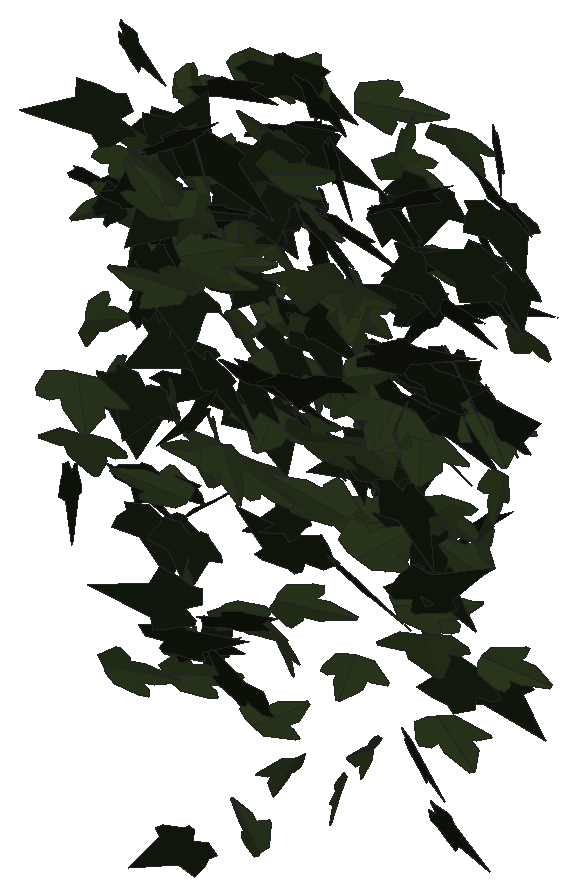
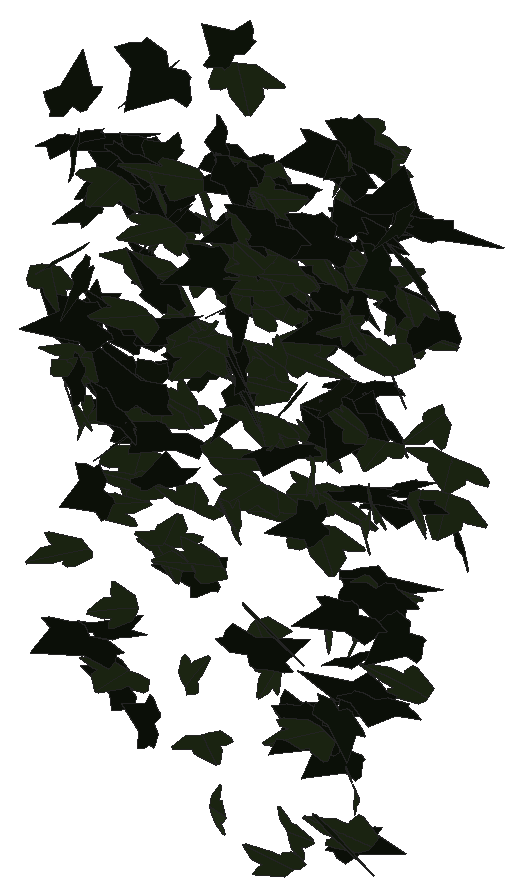
# SketchUp Ruby script. Lengths in millimetres.
U = 1.mm
M = Sketchup.active_model
def pt(a) = Geom::Point3d.new(a.map { |v| v * U })
def face(e, loops, mat)
  f = e.add_face(loops[0].map { |a| pt(a) })
  loops[1..].each { |l| e.add_face(l.map { |a| pt(a) }).erase! }
  f.material = f.back_material = mat if mat
  f
end
# faces: each face lists its corners as indices into pts; further lists are holes
def faces(e, pts, list, mat = nil) = list.each { |f| face(e, (f[0].is_a?(Array) ? f : [f]).map { |l| l.map { |i| pts[i] } }, mat) }
# xy, xz, yz: faces in a plane at the given z, y or x. An outline is a flat list of corners, or four numbers for a rectangle; further outlines are holes
def ring(l) = l.size == 4 ? [[l[0], l[1]], [l[2], l[1]], [l[2], l[3]], [l[0], l[3]]] : l.each_slice(2).to_a
def flat(e, list, mat, &to3) = list.each { |f| face(e, (f[0].is_a?(Array) ? f : [f]).map { |l| ring(l).map { |u, v| to3.(u, v) } }, mat) }
def xy(e, z, list, mat = nil) = flat(e, list, mat) { |x, y| [x, y, z] }
def xz(e, y, list, mat = nil) = flat(e, list, mat) { |x, z| [x, y, z] }
def yz(e, x, list, mat = nil) = flat(e, list, mat) { |y, z| [x, y, z] }
def lines(e, pts, list) = list.each { |a, b| e.add_line(pt(pts[a]), pt(pts[b])) }
# prism: a flat outline (further loops are holes) pulled along v
def prism(e, loops, v, mat = nil)
  f = face(e, loops, mat); d = Geom::Vector3d.new(v.map { |x| x * U })
  f.pushpull(f.normal.samedirection?(d) ? d.length : -d.length)
end
def box(e, o, s, mat = nil) = prism(e, [[o, [o[0] + s[0], o[1], o[2]], [o[0] + s[0], o[1] + s[1], o[2]], [o[0], o[1] + s[1], o[2]]]], [0, 0, s[2]], mat)
def at(x, y, z, deg = 0) = Geom::Transformation.translation(pt([x, y, z])) * Geom::Transformation.rotation(ORIGIN, Z_AXIS, deg.degrees)
def axes(o, x, y, z) = Geom::Transformation.new([*x, 0, *y, 0, *z, 0, *pt(o).to_a, 1])
def part(name) = M.definitions.add(name)
# library, detail: a bought-in or finely detailed component or shape, given as its bounding box
def library(name, o, s) = part(name).tap { |d| box(d.entities, o, s) }
def detail(e, o, s) = box(e.add_group.entities, o, s)
def put(e, d, t, mat = nil) = e.add_instance(d, t).tap { |i| i.material = mat if mat }
def group(e, t, mat = nil) = e.add_group.tap { |g| g.transformation = t; g.material = mat if mat }.entities
root = M.entities
M.materials.add("efeu1").color = [18, 25, 13]
M.materials.add("efeu2").color = [43, 57, 29]
c1 = part("ivyleaf_9")
p = [[39.1,54.8,31.7],[34.5,51.8,30.2],[-5.3,25.2,17.3],[-17.9,28.3,20.9],[-21.6,21.7,17],[-20.2,4.3,5.3],
  [-22.9,-0.3,2.5],[-17.1,-4,-0.6],[-2,-2.1,-1.2],[-0.7,-15.4,-10.1],[16.6,-22.3,-16.7],[21.1,-15.1,-12.5],
  [32.7,-10.7,-11],[46.1,-1.8,-6.6],[30.8,11.2,3.8]]
faces(c1.entities,p,[[0,1,2,3,4,5,6,7,8,9,10,11,12,13,14]],"efeu1")
c2 = part("ivyleaf_10")
p = [[0,12.8,-0.8],[-1.5,51.3,-10.9],[-4.9,51,-11.6],[-13.6,26.5,-7.3],[-13.2,15.9,-4.6],[-21.1,19.3,-7.2],
  [-29.5,16.3,-8.3],[-29.2,8.3,-6.2],[-19.7,-9.8,0.5],[-7.6,-13,4],[1,-12.2,5.8],[-0.4,51.1,-11.1],
  [-1.5,51.1,-10.9],[1,-12.4,5.9],[16.9,-12.4,3.5],[35.1,9.1,-5.1],[35,12.9,-6.1],[20.5,16.4,-4.9],
  [15.8,15,-3.8],[15.3,27.6,-7.1],[12.8,31.3,-7.8]]
faces(c2.entities,p,[[0,1,2,3,4,5,6,7,8,9,10],[11,12,0,13,14,15,16,17,18,19,20]],"efeu2")
put(root,c1,axes([4369.1,966.1,860.8],[0.08362,0.95421,0.22388],[0.01446,0.22376,-0.95522],[-1.86531,0.04451,0.00263]))
put(root,c1,axes([4349,904.5,861.4],[-1.16613,-0.65303,-0.50074],[0.6447,0.3688,-0.89547],[1.42733,-0.70011,-0.00464]))
put(root,c1,axes([4339.9,842.3,951.2],[1.8565,-0.13492,-0.2079],[-0.3923,0.02714,-0.98475],[0.26191,0.997,-0.00132]))
put(root,c2,axes([4325.6,979.6,1366.4],[0.13539,-0.04871,-0.98589],[1.45694,-0.62129,0.08593],[-1.18599,-0.76879,-0.00698]))
put(root,c1,axes([4331.7,974.3,1044],[-0.12536,-0.06032,-0.97559],[1.05105,0.80448,-0.08703],[1.53491,-0.55581,-0.02009]))
put(root,c2,axes([4353,806.8,1143],[0.80808,-0.87307,0.54689],[0.48755,-0.48346,-0.9707],[1.89912,0.49561,0.0165]))
put(root,c2,axes([4335.4,884.7,1433.3],[-1.12404,-0.39241,0.74969],[1.311,0.30801,0.70389],[-0.93531,0.90331,0.08566]))
put(root,c2,axes([4349,889.3,1289],[1.19402,0.76921,0.28156],[0.33803,0.21847,-0.99262],[-1.52186,0.65203,0.00042]))
put(root,c2,axes([4384.4,775.3,1420.2],[-0.29948,-0.47217,1.00902],[-0.61085,-0.95661,-0.4977],[2.03032,-0.35746,-0.0009]))
put(root,c1,axes([4406.1,733.1,1573.3],[-1.48282,-0.09995,0.76812],[-1.4335,-0.15652,-0.78436],[0.34408,-1.08284,0.04247]))
put(root,c1,axes([4359.3,816.4,1643.3],[1.15418,-0.58438,-0.50934],[-0.66761,0.36982,-0.84195],[1.31566,0.70031,0.01959]))
put(root,c1,axes([4399,966.8,661.1],[-1.38357,0.66362,0.05925],[-0.09114,0.03543,-0.98429],[-1.26474,-0.72852,0.00611]))
put(root,c1,axes([4366,757.4,1452.9],[1.98036,0.33777,-0.35353],[-0.63959,-0.10976,-1.09399],[-0.67593,1.09347,-0.0006]))
put(root,c2,axes([4361.9,940.6,1512.6],[0.30545,-0.11876,-0.96776],[0.94304,0.85462,-0.0227],[1.59816,-0.4816,0.19836]))
put(root,c2,axes([4355.6,949.9,1519],[1.05825,-0.44127,0.74741],[1.17973,-0.41942,-0.70877],[1.15626,0.83179,0.03911]))
put(root,c2,axes([4369.8,729.5,1255.1],[-0.17725,-0.40606,-1.14802],[0.83155,1.06357,-0.41164],[2.16325,-0.44211,0.06417]))
put(root,c2,axes([4397.7,896.8,685.7],[0.56411,-0.3148,0.91613],[-1.17037,0.67911,0.43231],[-1.42452,-0.68261,0.00761]))
put(root,c2,axes([4372.1,881.7,1179.1],[0.98885,-0.68468,0.48017],[0.63832,-0.34723,-0.85805],[1.45799,0.6164,0.05]))
put(root,c2,axes([4387.2,690.7,1090.6],[-2.02819,-0.35712,-0.10063],[0.18217,0.03107,-1.12392],[0.68223,-1.06997,0.00095]))
put(root,c2,axes([4370.3,695.8,1166.9],[2.24369,0.23405,0.24291],[0.45397,0.04596,-1.20191],[-0.45394,1.20279,-0.00134]))
put(root,c2,axes([4382.9,782.6,1482.1],[1.79201,-0.20378,0.04962],[0.09409,-0.00616,-0.96337],[0.38792,0.94286,0.00444]))
put(root,c1,axes([4365.8,969.4,1400],[0.87995,-0.91926,0.05132],[0.05251,-0.04357,-1.02897],[1.75148,0.46315,0.00506]))
put(root,c2,axes([4403.5,950.5,985.9],[0.23616,-0.08133,-0.97729],[-0.39029,0.96115,-0.10602],[1.82514,0.21606,0.10378]))
put(root,c1,axes([4376.9,675.4,1040],[-0.77384,0.16227,-1.11029],[1.91542,-0.46946,-0.43717],[-0.94432,-1.0852,0.0231]))
put(root,c1,axes([4380,844.5,1306.2],[-1.03249,-0.02704,-1.02633],[1.91792,-0.23601,-0.52646],[-0.37366,-1.13664,0.13373]))
put(root,c2,axes([4370.7,920,623.6],[-0.63526,-0.27157,0.93693],[1.32949,0.62466,0.42992],[-1.29588,0.77399,-0.01823]))
put(root,c1,axes([4415.4,820,988.4],[0.9954,0.51429,-0.71464],[-0.94926,-0.51191,-0.73343],[-1.38088,0.72263,-0.01096]))
put(root,c1,axes([4426.9,871.3,1175.7],[-1.62625,-0.49849,0.46439],[-0.7161,-0.27571,-0.98828],[1.08094,-0.93262,0.04394]))
put(root,c1,axes([4398.7,784.2,1128.4],[-1.05671,-0.93141,-0.33338],[0.31188,0.29043,-1.08432],[1.85679,-0.57886,-0.0076]))
put(root,c1,axes([4400.6,887.1,1322.5],[1.45418,0.83812,0.01786],[0.01517,0.0169,-1.13412],[-1.59541,0.76409,0.0055]))
put(root,c2,axes([4436.5,817.9,972.8],[0.49977,0.20311,0.97216],[-1.43079,-0.61645,0.33186],[1.23515,-0.79627,-0.00894]))
put(root,c1,axes([4416.3,885.7,1265.8],[1.82952,-0.16489,0.73967],[-1.37559,0.15964,0.97493],[-0.43354,-1.20237,0.028]))
put(root,c1,axes([4419.7,776,1143.9],[-0.89959,-0.91093,0.18622],[-0.14131,-0.17125,-1.02618],[1.76388,-0.4783,0.01276]))
put(root,c2,axes([4416.1,740.7,1438],[-1.3582,-0.55909,-0.43768],[0.6418,0.27921,-0.9065],[1.1892,-0.78923,-0.01065]))
put(root,c2,axes([4445.2,936.9,1230.9],[-0.05536,0.00098,0.98374],[-1.14119,0.7802,-0.0185],[-1.48426,-0.5999,-0.02246]))
put(root,c2,axes([4407.5,851.7,1096.6],[0.10695,-0.18999,1.00594],[1.29492,-0.74582,-0.17887],[1.45577,0.67737,0.0852]))
put(root,c1,axes([4426.3,781.2,1514.1],[0.48535,0.48483,0.93654],[0.70036,0.86207,-0.54647],[-1.88095,0.44608,0.03818]))
put(root,c1,axes([4420.9,698.2,1450.6],[-0.47481,0.97999,0.35571],[0.11532,-0.3515,1.0109],[1.98083,0.25537,0.02641]))
put(root,c1,axes([4432.4,857,886.2],[-0.51891,-0.94728,0.00725],[0.02076,-0.01069,-0.98564],[1.80279,-0.27254,0.01344]))
put(root,c1,axes([4412.7,962.1,1167.4],[1.54235,-0.56391,0.06856],[0.1066,-0.03954,-0.98729],[1.07587,0.81233,-0.00046]))
put(root,c1,axes([4458.6,727.2,1295.4],[0.01571,0.26816,1.04274],[-0.05132,1.04249,-0.26788],[-2.04847,-0.02406,0.01471]))
put(root,c1,axes([4420,882.8,1462.4],[-0.0388,-0.09909,-1.03263],[0.85389,0.93039,-0.09814],[1.78011,-0.44845,0.02457]))
put(root,c1,axes([4447.8,853.8,719.3],[1.00163,0.68671,0.54597],[0.66595,0.41953,-0.86498],[-1.53111,0.63171,-0.01905]))
put(root,c2,axes([4464.1,832.8,1455.6],[-0.2123,1.09921,-0.06423],[0.00569,-0.06426,-1.10485],[-2.09558,-0.11154,0.00351]))
put(root,c2,axes([4454.4,931.4,1191.2],[-0.85746,0.5092,-0.71379],[0.80663,-0.57605,-0.67845],[-1.46082,-0.61696,0.04435]))
put(root,c2,axes([4441,696.4,756],[-0.57566,-0.08255,0.97235],[1.71913,0.36153,0.31168],[-0.70279,0.95197,-0.03405]))
put(root,c1,axes([4467.7,787.4,1308.1],[-0.8331,-0.85574,-0.42712],[0.38793,0.37547,-0.96115],[1.77842,-0.48277,0.00957]))
put(root,c2,axes([4480.5,794.2,871.7],[0.00937,0.27558,-1.00343],[-0.03188,-1.00329,-0.27563],[-1.98019,0.01745,-0.00031]))
put(root,c2,axes([4454.1,959.7,1575.4],[1.08792,0.113,0.81816],[1.54398,0.10991,-0.58198],[-0.29499,0.992,-0.02872]))
put(root,c1,axes([4454.8,784.1,766.5],[0.35911,-0.03637,0.96057],[1.82761,-0.03699,-0.19003],[0.08246,0.97823,0.02852]))
put(root,c1,axes([4473.2,882.4,765.1],[1.51336,0.55938,0.31258],[0.4871,0.17945,-0.97221],[-1.11806,0.83534,-0.00047]))
put(root,c1,axes([4470.9,859.4,1589.3],[1.47334,0.50657,0.45417],[0.72328,0.24869,-0.92515],[-1.07402,0.86239,0]))
put(root,c1,axes([4492.4,764.9,1570.4],[-1.69255,-0.20314,-0.54791],[1.01965,0.11491,-0.9122],[0.44403,-1.03821,0.00624]))
put(root,c2,axes([4467.7,972,567.5],[1.01744,0.25007,-0.79473],[1.29696,0.412,0.58804],[0.91225,-0.86466,0.05035]))
put(root,c2,axes([4470.6,904,761.9],[-1.14061,-0.20053,-0.82563],[1.4739,0.28666,-0.63177],[0.66513,-0.97912,-0.01588]))
put(root,c2,axes([4532.5,875.4,1376],[0.465,0.09094,-1.01984],[-1.94865,0.02318,-0.24322],[0.00276,1.04844,0.09384]))
put(root,c1,axes([4493.6,762.7,1550.8],[-1.13016,-0.23025,0.85214],[1.50464,0.31805,0.63686],[-0.74719,0.98874,-0.00642]))
put(root,c2,axes([4519,828.2,1050.8],[-1.88062,-0.47344,0.28694],[-0.46015,-0.15906,-1.09505],[0.94783,-1.01659,0.0377]))
put(root,c1,axes([4521,749.3,496.3],[-0.01194,-0.12235,-0.99511],[0.08968,-0.99406,0.12193],[-1.90604,-0.046,0.01197]))
put(root,c2,axes([4544.4,777.6,1086.2],[0.89251,-0.09222,-0.95319],[-1.73618,0.27989,-0.47589],[0.55452,1.02477,0.04419]))
put(root,c1,axes([4514,661.7,1515.9],[1.50421,0.26559,0.76895],[-1.38324,-0.25115,0.83377],[0.69563,-1.07372,-0.00482]))
put(root,c1,axes([4554,689.7,894.6],[-0.88472,-0.0952,0.97458],[-1.82341,-0.17874,-0.47445],[0.38516,-1.06487,-0.00749]))
put(root,c1,axes([4531.6,715.4,1496.6],[-1.47401,-0.87377,0.45369],[-0.5399,-0.3547,-1.16741],[1.7943,-0.82453,0.02143]))
put(root,c2,axes([4504.5,817.4,1491.1],[1.92257,-0.55658,-0.25771],[0.43349,-0.12063,1.15335],[-1.08385,-1.03553,0.00415]))
put(root,c1,axes([4513.1,776.8,1448.4],[1.41254,0.74828,0.16011],[0.21525,0.11333,-1.05393],[-1.44036,0.75076,-0.00048]))
put(root,c2,axes([4537.3,811.7,1408.4],[1.18762,-0.65114,0.84942],[-1.1293,0.60784,0.90185],[-1.69525,-0.86107,-0.0057]))
put(root,c2,axes([4562.6,662.6,1397.6],[-0.7031,-0.22943,-1.12963],[-1.83305,-0.59027,0.43487],[-1.20528,1.03156,-0.0024]))
put(root,c2,axes([4519.9,962.3,1566],[1.25277,0.49314,-0.58738],[0.89368,0.35288,0.82248],[1.15409,-0.80856,0.00071]))
put(root,c1,axes([4569.2,922.1,939],[-1.52749,0.59372,-0.03443],[0.03889,-0.03028,-0.99825],[-1.13119,-0.80276,0.01218]))
put(root,c1,axes([4573,923.9,870.6],[0.43653,-0.00539,1.00933],[-1.83586,0.30352,0.22083],[-0.56548,-0.98956,0.06224]))
put(root,c1,axes([4565.5,814.5,702.2],[0.71666,-0.53585,0.84186],[-0.88975,0.70023,0.65481],[-1.67796,-0.60017,0.01234]))
put(root,c1,axes([4584.9,952.2,1387.8],[-0.28727,0.05194,-1.00048],[-1.75489,0.38841,0.15927],[0.74552,0.93429,-0.01059]))
put(root,c2,axes([4540.1,791,1369.3],[-0.20924,-0.10709,-1.14825],[1.4016,0.88112,-0.15269],[1.68903,-0.74444,-0.01554]))
put(root,c1,axes([4533.9,918.7,1612.5],[-0.22336,-0.13773,-1.1601],[1.2404,0.95992,-0.1799],[1.84526,-0.66194,-0.01949]))
put(root,c1,axes([4557.7,652.7,1625.4],[1.07682,0.85095,0.73106],[0.74731,0.61678,-1.02181],[-2.00007,0.6886,0.01181]))
put(root,c2,axes([4552.7,857.3,1498.1],[1.84675,0.32831,0.23338],[0.42588,0.06681,-1.02434],[-0.63745,0.99577,-0.00822]))
put(root,c2,axes([4537.8,893.2,1364.6],[0.23248,-0.22728,1.01631],[1.73827,-0.46827,-0.2145],[0.95229,0.91024,0.14342]))
put(root,c2,axes([4540.5,732.4,1388.1],[-0.57451,-0.26093,-1.05407],[1.74191,0.52759,-0.39272],[1.11212,-0.96116,0.07059]))
put(root,c2,axes([4595.6,799.2,501.4],[0.95298,-0.28781,0.93325],[-1.55861,0.44766,0.57745],[-1.01268,-0.95984,-0.01052]))
put(root,c2,axes([4564.2,707.9,1605],[-0.61669,1.14319,-0.35051],[0.15808,-0.34075,-1.18816],[-2.2702,-0.33427,0.01248]))
put(root,c2,axes([4606.7,596.6,1597.5],[-0.30657,0.12198,-1.11142],[-1.53328,0.76597,0.20083],[1.47556,0.82128,-0.02223]))
put(root,c1,axes([4549.8,966.3,1383],[0.27187,-0.06416,-1.00043],[1.72198,-0.42691,0.15657],[-0.82159,-0.91598,-0.0029]))
put(root,c1,axes([4574.5,831.6,1349.5],[-0.50524,-0.74929,0.72249],[-0.49624,-0.67398,-0.79478],[1.91784,-0.37178,-0.01531]))
put(root,c2,axes([4596.3,931.9,1598.1],[0.79519,-0.67196,-0.78138],[-0.80695,0.6564,-0.79121],[1.78769,0.59519,-0.00958]))
put(root,c2,axes([4597.6,599.9,1562.3],[1.71992,0.26235,0.6247],[-1.14988,-0.15932,0.94092],[0.58366,-1.08699,0.01286]))
put(root,c2,axes([4588.9,821.3,1405.9],[-0.83548,-0.74988,-0.66441],[-0.62713,-0.57697,0.86891],[-1.8007,0.54887,0.00566]))
put(root,c1,axes([4618.6,821,1440.7],[-0.74678,0.54894,0.83917],[-1.09236,0.61597,-0.67131],[-1.56493,-0.69192,0.06814]))
put(root,c2,axes([4558.7,973.9,1113.7],[-0.19709,0.11124,1.08707],[1.62323,-0.67439,0.15026],[1.30012,0.85886,-0.02281]))
put(root,c1,axes([4571.2,814,1481.1],[-0.39585,-0.76517,-0.84013],[0.52369,0.79476,-0.79197],[2.09835,-0.3427,0.03916]))
put(root,c1,axes([4596.3,859.7,1570.5],[1.00952,1.01229,-0.1151],[-0.10076,-0.1022,-1.14284],[-1.93638,0.53307,-0.00054]))
put(root,c1,axes([4577.2,855.2,1536.9],[0.02248,-0.66751,0.82208],[0.30504,-0.81153,-0.66125],[1.99219,0.13179,0.09197]))
put(root,c2,axes([4599,840.6,796.6],[-1.27629,0.74452,-0.04122],[0.04466,-0.03433,-1.00199],[-1.41844,-0.67099,0.00554]))
put(root,c2,axes([4599.5,656.8,1525],[-0.19401,-0.82834,-0.8697],[0.52612,0.83321,-0.82599],[2.22447,-0.26931,0.11951]))
put(root,c2,axes([4600.1,811.5,1512.6],[0.57575,-0.79694,0.60526],[0.38159,-0.57123,-0.85234],[1.86598,0.36271,-0.01245]))
put(root,c1,axes([4625.7,874.4,1268.4],[-0.03725,0.48991,1.15271],[-0.21639,1.1474,-0.48958],[-2.37392,-0.11227,0.02654]))
put(root,c2,axes([4638.1,806.2,1572.9],[-0.99659,0.1837,-0.84799],[-1.53731,0.25843,0.55478],[0.60295,0.96254,0.01288]))
put(root,c2,axes([4576.9,847.7,1285.7],[0.61891,0.0119,-0.99694],[1.64994,0.51451,0.28893],[0.93713,-0.91373,0.14971]))
put(root,c1,axes([4598.4,814.9,1162],[-0.49934,-1.03759,-0.42875],[0.17198,0.41936,-1.07016],[2.12976,-0.27713,-0.01411]))
put(root,c2,axes([4577.4,687.4,1445],[1.39699,-0.27168,-0.86308],[1.58409,-0.23316,0.78126],[-0.67543,-1.10875,0.04719]))
put(root,c1,axes([4578.3,695.5,1610.3],[-0.33903,-0.08069,-1.29109],[2.29001,0.46823,-0.19528],[0.90405,-1.21631,0.01048]))
put(root,c2,axes([4582.3,804.4,1056.2],[0.93363,0.06294,0.91802],[1.67448,0.27263,-0.48884],[-0.51295,1.00453,0.07515]))
put(root,c2,axes([4617.1,844.3,1222.4],[2.16021,0.14642,-0.02052],[-0.03913,-0.00104,-1.14444],[-0.27865,1.13522,0.0016]))
put(root,c1,axes([4614,759.6,1226.7],[0.92057,-0.56875,-0.69273],[-0.77994,0.55973,-0.7457],[1.51709,0.63288,0.03698]))
put(root,c2,axes([4609.8,871.6,1117.9],[-1.59822,-0.23423,-0.58337],[1.05167,0.18912,-0.87136],[0.57047,-1.00486,-0.02801]))
put(root,c2,axes([4598.8,721.7,1127.4],[1.54951,-0.35343,0.68704],[1.20748,-0.26378,-0.88753],[0.83918,1.03214,0.00844]))
put(root,c1,axes([4600.9,686.3,1283.6],[1.02195,-1.07695,-0.0969],[-0.08037,0.08722,-1.20339],[2.05636,0.53862,0.00112]))
put(root,c2,axes([4631.8,832.9,1542.7],[-0.52334,-0.6853,-0.78542],[-0.27845,-0.77887,0.73081],[-1.96419,0.29301,0.10566]))
put(root,c1,axes([4649.2,868.8,1370],[0.20281,-0.42793,1.17445],[0.02401,1.17902,0.42845],[-2.37885,-0.02458,0.10445]))
put(root,c2,axes([4635.6,955.3,717.6],[1.20365,0.71801,-0.31985],[-0.43122,-0.22658,-0.95663],[-1.43248,0.67152,0.01922]))
put(root,c2,axes([4600.8,855.3,1452.6],[0.77909,0.15052,0.95337],[1.67494,0.367,-0.43582],[-0.75424,0.97046,0.01695]))
put(root,c2,axes([4636.2,778.4,1174.6],[1.98133,0.05624,-0.12869],[-0.24512,-0.00155,-1.04256],[-0.10659,1.04897,0.00536]))
put(root,c2,axes([4654.1,803.2,1560.6],[1.3694,-0.81204,-0.51588],[-0.59429,0.4122,-1.08436],[1.73184,0.78354,0.03581]))
put(root,c1,axes([4657.5,854.1,1638.4],[1.05651,0.03019,-0.85806],[-1.62966,0.09444,-0.55065],[0.11989,1.0176,0.07656]))
put(root,c2,axes([4643.9,969.9,1119],[1.92212,0.09858,0.09952],[-0.20081,0.05895,1.01242],[0.17535,-1.01312,0.06859]))
put(root,c1,axes([4625.4,771.3,1583.6],[0.12687,-0.71013,-0.93458],[0.42673,0.92655,-0.68804],[2.19277,-0.13923,0.18797]))
put(root,c2,axes([4647.5,860.7,1345.3],[1.76522,0.41243,0.00353],[-0.00193,0.01098,-1.01501],[-0.78497,0.92744,0.01044]))
put(root,c2,axes([4657.8,899.6,565.2],[0.51674,-0.58831,0.83544],[0.72757,-0.74316,-0.64757],[1.80344,0.46838,0.02188]))
put(root,c2,axes([4676.6,762.7,1349.2],[-0.07597,-0.18331,1.05805],[0.00708,-1.0588,-0.1833],[2.04368,-0.00315,0.03997]))
put(root,c1,axes([4702.3,552.5,1310.1],[-1.24203,0.81064,-0.47546],[0.57246,-0.36823,-1.04068],[-1.69452,-0.71858,-0.00308]))
put(root,c1,axes([4654,800.6,1595.3],[0.2512,-0.21575,-1.14344],[1.08947,1.01393,-0.12524],[1.92808,-0.54482,0.21974]))
put(root,c2,axes([4669.2,760.8,1564.7],[-0.98719,-0.29308,0.90553],[1.49588,0.4497,0.59576],[-1.02157,0.9417,-0.00268]))
put(root,c2,axes([4667,905,982.2],[0.67892,0.05065,1.00626],[1.69691,0.48126,-0.3403],[-0.89301,0.953,0.11837]))
put(root,c2,axes([4699.6,879.2,1318],[-1.20997,-0.59603,-0.60846],[0.93498,0.36365,-0.86953],[1.32424,-0.80135,0.05798]))
put(root,c2,axes([4745.1,772.5,1076.1],[0.85229,0.28826,1.04519],[-1.7311,-0.51558,0.53191],[1.12305,-1.01348,0.02669]))
put(root,c1,axes([4683.8,853.2,1458],[1.88133,-0.23007,0.12023],[0.21974,-0.0343,-1.0149],[0.44249,0.9952,-0.00718]))
put(root,c1,axes([4696.9,959.9,1219.5],[-0.60373,-0.48965,-0.84121],[0.9957,0.6603,-0.58164],[1.56211,-0.61013,0.04563]))
put(root,c2,axes([4732.7,752.7,1342.6],[-1.06238,-0.64537,-0.57934],[-0.68213,-0.45572,0.85299],[-1.50302,0.66299,0.02237]))
put(root,c1,axes([4713.7,758.1,1189.1],[1.59995,-0.43945,-0.68809],[-1.09577,0.38117,-0.94685],[1.10172,1.0173,0.05754]))
put(root,c1,axes([4709.9,720.8,1334.9],[-0.14382,-0.90683,0.49811],[0.00905,-0.49973,-0.90906],[1.96907,-0.06394,0.04056]))
put(root,c1,axes([4694.1,654.8,1321.6],[2.365,-0.12436,0.23053],[0.43694,-0.02103,-1.24885],[0.24002,1.26367,0.00191]))
put(root,c2,axes([4734.3,831.4,1311],[0.2566,0.58742,-0.99],[0.21812,0.98497,0.60004],[2.18,-0.16769,0.05649]))
put(root,c2,axes([4737.2,913.6,1003.3],[1.30966,0.79262,0.05381],[-0.06708,-0.04067,1.04966],[1.51051,-0.68904,-0.00004]))
put(root,c1,axes([4703.1,853.2,927.4],[1.28894,-0.66916,0.44254],[0.60451,-0.30817,-0.95207],[1.4021,0.74803,0.00366]))
put(root,c1,axes([4724.6,763.6,1348.8],[0.26268,-1.12937,-0.07509],[-0.01514,0.07467,-1.13777],[2.15411,0.13824,0.00116]))
put(root,c2,axes([4755.1,668.9,734.1],[-0.37176,-1.08173,0.13943],[-0.03866,-0.13802,-1.09921],[2.07542,-0.19634,0.0045]))
put(root,c2,axes([4709.1,906.7,1627.2],[0.04588,-0.14888,-1.18285],[2.1689,0.35037,-0.02088],[0.66642,-1.13003,0.14937]))
put(root,c1,axes([4708.9,741.8,1385.8],[0.21144,-0.09159,-1.13251],[2.10344,0.27269,0.08637],[0.50165,-1.10479,0.11521]))
put(root,c2,axes([4754.2,905.7,978.9],[1.91999,-0.37496,-0.0712],[-0.12756,0.02404,-1.07625],[0.71508,1.01104,-0.00081]))
put(root,c2,axes([4737.3,922.9,1537.7],[-1.21856,-0.20766,-0.7731],[1.44661,0.15286,-0.67055],[0.47795,-0.9921,0.0585]))
put(root,c1,axes([4789.2,915.1,1336.3],[-0.22754,-0.01736,1.01393],[-1.72395,-0.45718,-0.11464],[0.86771,-0.91288,0.03813]))
put(root,c1,axes([4740,776.1,1618.3],[-0.11755,0.05022,-1.17516],[2.07158,-0.44358,-0.07616],[-0.84847,-1.08997,-0.02315]))
put(root,c2,axes([4761.7,902,1572.3],[1.18252,-0.80112,0.11044],[-0.11423,0.09321,1.01378],[-1.53486,-0.62415,0.00964]))
put(root,c1,axes([4776.7,883.4,1074.3],[-1.22661,-0.56207,0.64956],[1.03462,0.36185,0.8525],[-1.26577,0.84045,0.06736]))
put(root,c2,axes([4734.8,779.9,1411],[-0.45417,-0.13511,1.13339],[2.13223,0.19375,0.25898],[-0.41551,1.14192,0.09016]))
put(root,c2,axes([4783.1,768.4,1280.8],[1.71095,-0.72337,-0.15791],[-0.21722,0.11002,-1.1538],[1.3923,0.90609,0.01403]))
put(root,c2,axes([4784.4,806.8,702.1],[-0.18988,-0.23968,-0.99069],[-0.39434,-0.96988,0.25551],[-1.89938,0.22532,0.046]))
put(root,c1,axes([4776.4,842.1,1514.1],[0.74857,-0.57498,-0.76227],[-0.6751,0.67741,-0.694],[1.68713,0.52618,0.06051]))
put(root,c2,axes([4753.5,836.8,1186.2],[0.44385,-0.1254,1.09647],[1.96136,-0.37623,-0.26222],[0.75152,1.05598,0.03678]))
put(root,c2,axes([4767.3,949.5,1390.7],[-1.17826,0.0106,-0.8286],[1.56764,-0.1054,-0.61677],[-0.17272,-1.02895,0.05464]))
put(root,c1,axes([4779.1,898.5,668.7],[0.51927,-0.07466,-1.03772],[1.86212,-0.34636,0.28217],[-0.67326,-1.01555,-0.01994]))
put(root,c1,axes([4794.9,968.1,1234.3],[-0.91057,-0.01674,-1.01868],[1.93558,-0.07482,-0.47643],[-0.11539,-1.12295,0.04693]))
put(root,c1,axes([4795.9,744.4,1184.6],[0.07139,-0.82037,0.70868],[0.25133,-0.70037,-0.81773],[2.04786,0.11455,0.07565]))
put(root,c2,axes([4809.8,924.4,867],[0.21613,-0.2095,1.0564],[0.11649,1.06179,0.20399],[-2.04638,0.03832,0.12319]))
put(root,c1,axes([4801.1,914.7,1217.4],[-1.01345,0.01344,1.06052],[1.69294,-0.64061,0.45475],[1.0993,0.99893,0.27737]))
put(root,c2,axes([4818.5,943.8,1596.7],[-1.84857,0.14122,-0.33525],[0.62524,-0.07001,-0.98129],[-0.29736,-1.02514,0.02083]))
put(root,c2,axes([4839.3,705.7,1471.4],[0.6881,-0.89247,-0.6503],[-0.43576,0.60881,-0.96283],[2.05595,0.42774,0.01358]))
put(root,c1,axes([4856.8,751.3,1197.6],[-1.30906,-0.42722,0.7466],[-1.2196,-0.38321,-0.80965],[1.09212,-0.94003,-0.00925]))
put(root,c2,axes([4836.5,742.6,1239.1],[-1.55649,0.6453,0.02239],[-0.03549,0.01252,-1.04176],[-1.22837,-0.81804,0.00172]))
put(root,c1,axes([4814.8,843.1,1208.3],[1.70649,-0.74125,0.04984],[0.07584,-0.03001,-1.16336],[1.41189,0.89753,0.00226]))
put(root,c2,axes([4831.7,714.1,1337.9],[-0.05293,-0.01796,-1.04879],[1.20261,0.83714,-0.03109],[1.59347,-0.6324,-0.01137]))
put(root,c2,axes([4858.4,716.3,1237.5],[-1.77896,-0.62216,-0.26632],[0.42179,0.14768,-1.12285],[1.21699,-0.96063,-0.00013]))
put(root,c1,axes([4886.8,896.9,787.5],[-1.64308,-0.62694,0.10491],[0.17174,0.05427,1.06691],[-1.19753,0.86798,0.00907]))
put(root,c1,axes([4860.6,953.9,1436.4],[1.21917,-0.4603,-0.81916],[-1.26294,0.48029,-0.78881],[1.26609,0.92233,0.00195]))
put(root,c2,axes([4891.3,881.3,994.3],[1.18014,0.26001,0.85246],[-1.49083,-0.33632,0.67238],[0.80902,-0.99904,-0.00448]))
put(root,c1,axes([4841.8,790.4,1558],[0.36497,-0.77719,0.6517],[0.31954,-0.62977,-0.80044],[1.90372,0.2547,0.00941]))
put(root,c1,axes([4866.7,832.8,1576.5],[-1.64476,-0.16121,-0.56136],[1.04139,0.12708,-0.87887],[0.38868,-1.02266,-0.02073]))
put(root,c2,axes([4844.9,886.4,725.7],[1.64452,0.39509,0.51358],[0.88707,0.2157,-0.95012],[-0.8567,0.98177,0.00207]))
put(root,c1,axes([4848.9,951.4,1347.6],[1.29788,0.32679,0.71701],[1.24373,0.29527,-0.75611],[-0.83793,0.94444,-0.0117]))
put(root,c1,axes([4888.9,531.5,1429.3],[1.04938,0.9579,-0.36912],[-0.34631,-0.32117,-1.10525],[-1.92281,0.58062,-0.00239]))
put(root,c1,axes([4843.3,866,1229.5],[-0.02857,-0.08732,-1.18105],[2.21181,0.22615,-0.03149],[0.43362,-1.15929,0.08282]))
put(root,c2,axes([4856.1,709.8,1077.8],[1.42917,0.30671,-0.81484],[1.33475,0.42455,0.80612],[0.98192,-1.02353,0.0902]))
put(root,c1,axes([4852,843.2,1270],[-0.10646,0.05472,1.03283],[1.39317,-0.72862,0.07825],[1.39062,0.73415,0.00067]))
put(root,c2,axes([4896.3,544.9,1580.5],[-1.58572,-0.80668,0.12408],[-0.16985,-0.08621,-1.15972],[1.54402,-0.83795,-0.00014]))
put(root,c1,axes([4878.6,895.8,1030.3],[0.51915,0.51636,0.92297],[0.91048,0.78984,-0.58326],[-1.79512,0.54994,-0.02891]))
put(root,c2,axes([4862.3,585.1,1299.2],[-1.36681,-0.37332,0.86791],[1.73049,0.02311,0.76231],[-0.48857,1.12627,0.27204]))
put(root,c1,axes([4936.8,753.4,1097.9],[-0.814,0.01596,-1.11731],[-2.12261,0.06797,0.4279],[0.13167,1.19445,-0.00942]))
put(root,c1,axes([4875.9,745.6,1287.4],[-0.07046,0.04644,1.00377],[0.91508,-0.88118,0.0585],[1.67928,0.48213,0.01023]))
put(root,c2,axes([4870.5,712.8,1255.2],[-0.38157,0.06855,1.0293],[1.93334,-0.16936,0.20914],[0.34168,1.03488,-0.03396]))
put(root,c2,axes([4922.2,901.5,1229.7],[1.56967,0.19861,-0.59841],[-1.10494,-0.1451,-0.84832],[-0.46806,1.00859,-0.00421]))
put(root,c2,axes([4877.9,519.4,1090.8],[-0.58227,-0.18891,-1.10884],[1.78067,0.59512,-0.35954],[1.1883,-0.98436,-0.00457]))
put(root,c1,axes([4880.9,927.2,794.2],[-0.50912,-0.26465,-1.02395],[1.38337,0.72121,-0.3763],[1.4621,-0.77453,-0.00052]))
put(root,c1,axes([4883.4,576.9,1634.8],[0.36362,-0.89981,0.77544],[0.49493,-0.73467,-0.91657],[2.20586,0.31317,0.07783]))
put(root,c1,axes([4893.1,939.1,1618.4],[0.09535,-0.05438,-1.04227],[1.63799,-0.58813,0.07206],[-1.12366,-0.86195,0.0166]))
put(root,c1,axes([4895,739.1,1513.7],[1.07617,0.56557,0.84246],[1.13418,0.59548,-0.79975],[-1.56302,0.82151,-0.00028]))
put(root,c2,axes([4882.8,767.8,979.4],[0.67416,-0.11,-1.10319],[1.93015,0.50003,0.27578],[0.85242,-1.04521,0.24803]))
put(root,c2,axes([4898.4,791.7,1123.9],[-1.55674,-0.29092,-0.79368],[1.45323,0.21954,-0.8674],[0.69023,-1.11839,0.03619]))
put(root,c1,axes([4895.1,925.2,1226.4],[0.23323,-0.07194,-1.03317],[1.85061,-0.35018,0.13972],[-0.67859,-0.97971,0.02593]))
put(root,c1,axes([4920.4,689.8,1645.2],[1.14548,0.96743,0.61569],[0.53617,0.54929,-1.13849],[-2.11557,0.66303,0.04483]))
put(root,c1,axes([4900.9,677.9,1409.2],[0.5902,0.6953,-0.87256],[0.55571,0.82349,0.75997],[2.0494,-0.42353,0.04521]))
put(root,c1,axes([4943.1,739.7,1461],[-0.51901,0.53975,-0.86231],[0.72,-0.77493,-0.60469],[-1.79728,-0.46631,0.00677]))
put(root,c1,axes([4921.7,935.3,1426.6],[-0.00996,-1.02268,0.22363],[-0.04585,-0.22346,-1.02245],[1.99182,-0.01026,-0.02242]))
put(root,c1,axes([4956.4,822.7,1267.5],[0.02833,-0.70606,0.94235],[-0.0988,0.94111,0.70595],[-2.23886,-0.05046,-0.01923]))
put(root,c1,axes([4905.5,802,646.3],[0.53141,-0.00862,-0.99705],[1.88627,-0.11084,0.27851],[-0.20754,-1.02946,-0.02164]))
put(root,c1,axes([4929.5,752.6,1051.8],[0.82413,-0.83333,-0.55624],[-0.39601,0.51796,-0.93796],[1.86527,0.47815,0.04663]))
put(root,c2,axes([4949.2,748,1146.5],[-0.89302,-0.78123,-0.43289],[0.41172,0.37502,-0.91128],[1.64922,-0.51664,-0.0069]))
put(root,c2,axes([4936.6,866.7,1232.1],[1.48668,0.73417,0.24902],[0.35184,0.16692,-1.072],[-1.43291,0.80271,-0.00485]))
put(root,c2,axes([4953.1,637,1354],[1.89771,0.44571,-0.27095],[-0.47628,-0.10408,-1.09218],[-0.871,1.02802,0.00689]))
put(root,c2,axes([4973,900.8,1366.9],[-1.62798,0.2797,0.52223],[-0.93431,0.17874,-0.89983],[-0.6311,-0.98614,-0.01498]))
put(root,c2,axes([4956.7,708.6,974.9],[-1.90337,-0.64818,-0.21116],[0.33955,0.11296,-1.19177],[1.2522,-1.01588,0.0022]))
put(root,c1,axes([4933.1,838,1473.1],[1.2414,-0.79795,-0.17464],[-0.20901,0.1358,-1.03062],[1.54049,0.66145,0.00091]))
put(root,c2,axes([4967,641.8,1331.3],[-0.02124,-0.01002,1.08265],[-0.8169,0.99404,0.00478],[-1.89175,-0.42913,-0.01422]))
put(root,c2,axes([4951,871.1,1144.6],[1.33031,-0.74224,0.39536],[0.51087,-0.29029,-1.01955],[1.51681,0.74875,-0.00336]))
put(root,c2,axes([4977,806,1091],[-0.14127,0.16774,1.11083],[-0.95133,0.99205,-0.1832],[-1.91478,-0.50526,0.00907]))
put(root,c1,axes([4939.5,709.3,1035.3],[-0.03162,-0.00892,1.2084],[2.09009,0.50417,0.01882],[-0.95969,1.09832,0.00117]))
put(root,c1,axes([4943.3,736.5,1484.6],[2.18128,-0.0548,-0.0431],[-0.08041,0.01862,-1.1473],[0.10555,1.14677,0.01657]))
put(root,c2,axes([4967.7,681.5,1296.2],[2.07157,0.41556,0.02504],[0.04043,0.01456,-1.16508],[-0.7913,1.08866,0.00602]))
put(root,c1,axes([5010.3,774.9,1525.8],[-0.63144,-0.86753,-0.57155],[-0.36974,-0.5376,0.92877],[-1.94233,0.38436,0.00901]))
put(root,c1,axes([4956.1,856.2,1247.6],[-0.24773,-0.00362,1.19027],[1.06915,-1.05581,0.05822],[1.99716,0.56476,0.11648]))
put(root,c2,axes([4963,852.9,879.8],[0.4477,0.44206,0.95037],[0.89044,0.82731,-0.50062],[-1.78508,0.52355,-0.01137]))
put(root,c1,axes([4975,842.9,1577.4],[-0.20616,-1.02535,-0.37043],[0.06937,0.36864,-1.03105],[2.07373,-0.11427,-0.00234]))
put(root,c1,axes([4988.3,666.2,1569.7],[0.67608,-0.81068,-0.76645],[0.59287,-0.70029,0.88509],[-2.03882,-0.47246,0.00322]))
put(root,c1,axes([4990.5,822.6,1619],[1.52667,-0.78356,-0.41859],[0.56993,-0.29247,1.12135],[-1.59177,-0.85623,0.00003]))
put(root,c1,axes([4989,621.1,1249.3],[-0.91305,-0.01407,-1.09963],[2.09237,0.02302,-0.47994],[0.05087,-1.1995,0.00368]))
